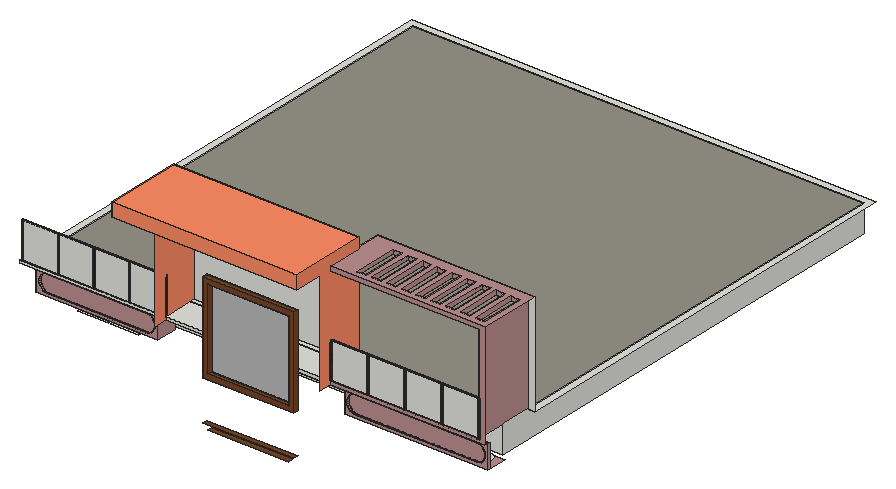
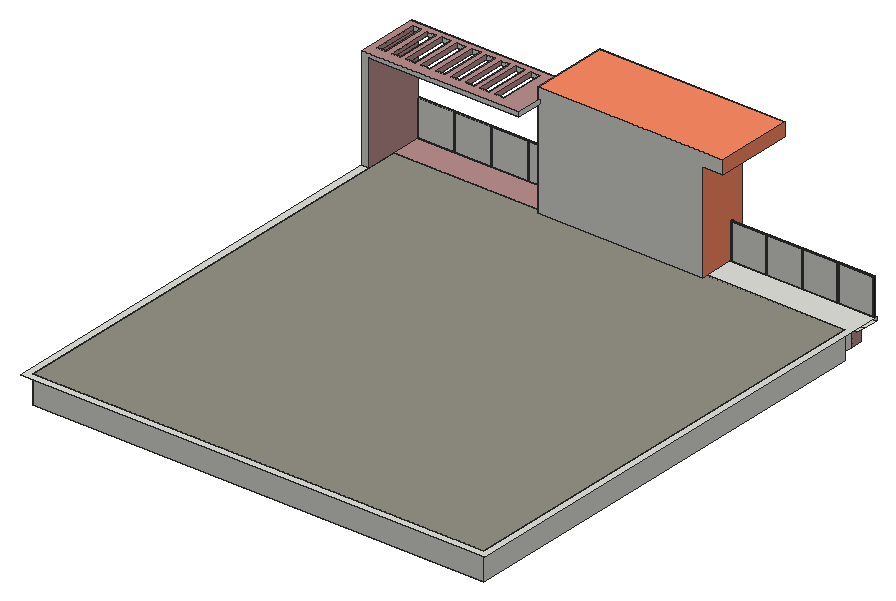
# SketchUp Ruby script. Lengths in inches.
U = 1.inch
M = Sketchup.active_model
def pt(a) = Geom::Point3d.new(a.map { |v| v * U })
def face(e, loops, mat)
  f = e.add_face(loops[0].map { |a| pt(a) })
  loops[1..].each { |l| e.add_face(l.map { |a| pt(a) }).erase! }
  f.material = f.back_material = mat if mat
  f
end
# faces: each face lists its corners as indices into pts; further lists are holes
def faces(e, pts, list, mat = nil) = list.each { |f| face(e, (f[0].is_a?(Array) ? f : [f]).map { |l| l.map { |i| pts[i] } }, mat) }
# xy, xz, yz: faces in a plane at the given z, y or x. An outline is a flat list of corners, or four numbers for a rectangle; further outlines are holes
def ring(l) = l.size == 4 ? [[l[0], l[1]], [l[2], l[1]], [l[2], l[3]], [l[0], l[3]]] : l.each_slice(2).to_a
def flat(e, list, mat, &to3) = list.each { |f| face(e, (f[0].is_a?(Array) ? f : [f]).map { |l| ring(l).map { |u, v| to3.(u, v) } }, mat) }
def xy(e, z, list, mat = nil) = flat(e, list, mat) { |x, y| [x, y, z] }
def xz(e, y, list, mat = nil) = flat(e, list, mat) { |x, z| [x, y, z] }
def yz(e, x, list, mat = nil) = flat(e, list, mat) { |y, z| [x, y, z] }
def lines(e, pts, list) = list.each { |a, b| e.add_line(pt(pts[a]), pt(pts[b])) }
# prism: a flat outline (further loops are holes) pulled along v
def prism(e, loops, v, mat = nil)
  f = face(e, loops, mat); d = Geom::Vector3d.new(v.map { |x| x * U })
  f.pushpull(f.normal.samedirection?(d) ? d.length : -d.length)
end
def box(e, o, s, mat = nil) = prism(e, [[o, [o[0] + s[0], o[1], o[2]], [o[0] + s[0], o[1] + s[1], o[2]], [o[0], o[1] + s[1], o[2]]]], [0, 0, s[2]], mat)
def at(x, y, z, deg = 0) = Geom::Transformation.translation(pt([x, y, z])) * Geom::Transformation.rotation(ORIGIN, Z_AXIS, deg.degrees)
def axes(o, x, y, z) = Geom::Transformation.new([*x, 0, *y, 0, *z, 0, *pt(o).to_a, 1])
def part(name) = M.definitions.add(name)
# library, detail: a bought-in or finely detailed component or shape, given as its bounding box
def library(name, o, s) = part(name).tap { |d| box(d.entities, o, s) }
def detail(e, o, s) = box(e.add_group.entities, o, s)
def put(e, d, t, mat = nil) = e.add_instance(d, t).tap { |i| i.material = mat if mat }
def group(e, t, mat = nil) = e.add_group.tap { |g| g.transformation = t; g.material = mat if mat }.entities
root = M.entities
M.materials.add("[0119_RosyBrown]").color = [188, 143, 143]
M.materials.add("[0136_Charcoal]").color = [35, 35, 35]
M.materials.add("[Color B03]").color = [255, 140, 101]
M.materials.add("[Formica Graystone]").color = [149, 146, 135]
M.materials.add("[Mirror 01]").color = [185, 185, 185]
M.materials.add("[Wood Veneer 01]").color = [120, 70, 37]
c1 = part("Group\#2")
box(c1.entities,[-152.36,0,0],[152.36,1.57,1.57])
c2 = part("Glass+Wall")
g1 = group(c2.entities,at(79.73,0,0))
g2 = group(g1,at(0,0,0))
g3 = group(g2,at(195.28,0,0),"[0136_Charcoal]")
box(g3,[-195.28,0,0],[195.28,1.57,1.57])
put(g2,c1,axes([1.57,0,116.54],[0,0,0.75452],[0,1,0],[-1,0,0]),"[0136_Charcoal]")
put(g2,c1,axes([50,0,116.54],[0,0,0.75452],[0,1,0],[-1,0,0]),"[0136_Charcoal]")
g4 = group(g2,at(195.28,0,115.75),"[0136_Charcoal]")
box(g4,[-195.28,0,0.79],[195.28,1.57,1.57])
put(g2,c1,axes([98.43,0,116.54],[0,0,0.75452],[0,1,0],[-1,0,0]),"[0136_Charcoal]")
put(g2,c1,axes([146.85,0,116.54],[0,0,0.75452],[0,1,0],[-1,0,0]),"[0136_Charcoal]")
put(g2,c1,axes([195.28,0,116.54],[0,0,0.75452],[0,1,0],[-1,0,0]),"[0136_Charcoal]")
g5 = group(g1,at(1.57,0.39,1.57))
box(g5,[0,0,0],[192.125,0.79,114.96])
xy(root,532.24,[[376.4,74.37,481.09,80.37]],"[Wood Veneer 01]")
xy(root,538.24,[[370.4,74.37,487.09,80.37]],"[Wood Veneer 01]")
xy(root,582.67,[[177.8,113.37,216.8,116.37],[219.92,113.37,255.8,116.37]])
xy(root,585.67,[[174.8,113.37,258.8,116.37]])
xy(root,590.49,[[370.4,74.37,487.09,80.37]],"[Wood Veneer 01]")
xy(root,595.17,[[593.68,113.37,630.53,116.37],[633.47,113.37,667.37,116.37]])
xy(root,596.49,[[376.4,74.37,481.09,80.37]],"[Wood Veneer 01]")
xy(root,598.17,[[590.68,113.37,670.37,116.37]])
xy(root,600,[[134.37,125.37,716.37,707.37]])
xy(root,602,[[540.59,89.37,725.37,92.37],[540.59,92.37,725.37,116.37]],"[0119_RosyBrown]")
xy(root,602.86,[[142.36,89.37,299.74,116.37]],"[0119_RosyBrown]")
xy(root,603.1875,[[291.4,94.48,293.11,94.75,294.69,95.46,296.04,96.55,297.05,97.95,297.67,99.56,297.85,101.28,297.58,102.99,296.88,104.57,295.79,105.91,294.39,106.93,292.78,107.55,291.06,107.73,289.35,107.46,287.77,106.76,286.42,105.67,285.41,104.27,284.79,102.65,284.61,100.93,284.88,99.23,285.58,97.65,286.67,96.3,288.07,95.28,289.68,94.66]])
xy(root,603.5,[[152.5,94.42,154.24,94.59,155.875,95.2,157.3,96.21,158.41,97.56,159.13,99.14,159.42,100.87,159.26,102.6,158.65,104.24,157.64,105.66,156.29,106.77,154.7,107.5,152.98,107.79,151.24,107.625,149.61,107.01,148.18,106,147.07,104.66,146.35,103.07,146.06,101.35,146.22,99.61,146.83,97.97,147.84,96.55,149.19,95.4375,150.78,94.71]])
xy(root,605,[[552.4375,89.37,712.19,92.37]],"[0119_RosyBrown]")
xy(root,605.86,[[153.74,89.37,288.27,92.37]])
xy(root,607.5,[[714.7,95.41,716.49,95.64,718.16,96.33,719.6,97.4375,720.7,98.875,721.4,100.55,721.63,102.34,721.4,104.14,720.7,105.8125,719.6,107.25,718.16,108.35,716.49,109.04,714.7,109.28,712.9,109.04,711.23,108.35,709.79,107.25,708.6875,105.8125,707.99,104.14,707.76,102.34,707.99,100.55,708.6875,98.875,709.79,97.4375,711.23,96.33,712.9,95.64]])
xy(root,621.125,[[548.88,95.41,550.68,95.64,552.35,96.33,553.79,97.4375,554.89,98.875,555.58,100.55,555.82,102.34,555.58,104.14,554.89,105.8125,553.79,107.25,552.35,108.35,550.68,109.04,548.88,109.28,547.09,109.04,545.41,108.35,543.98,107.25,542.875,105.8125,542.18,104.14,541.95,102.34,542.18,100.55,542.875,98.875,543.98,97.4375,545.41,96.33,547.09,95.64]])
xy(root,623,[[321.71,104.37,516.05,116.37]])
xy(root,629,[[153.74,89.37,288.27,92.37],[552.4375,89.37,712.19,92.37]],"[0119_RosyBrown]")
xy(root,632,[[125.37,85.68,142.36,104.37],[142.36,85.68,299.74,89.37],[299.74,85.68,312.71,89.37],[312.71,85.68,525.05,89.37],[525.05,85.68,725.37,89.37],
  [142.36,89.37,299.74,116.37],[299.74,89.37,312.71,116.37],[312.71,89.37,525.05,104.37],[525.05,89.37,540.59,116.37],[540.59,89.37,725.37,92.37],
  [125.37,104.37,142.36,116.37]])
xy(root,636,[[125.37,85.68,312.71,85.68,312.71,125.37,134.37,125.37,134.37,707.37,716.37,707.37,716.37,165.62,725.37,165.62,725.37,716.37,125.37,716.37],[312.71,85.68,525.05,125.37],[312.71,125.37,525.05,131.99]])
xy(root,636,[[525.05,85.68,716.37,125.37]],"[0119_RosyBrown]")
xy(root,636,[[134.37,125.37,312.71,125.37,312.71,131.99,525.05,131.99,525.05,125.37,716.37,125.37,716.37,707.37,134.37,707.37]],"[Formica Graystone]")
xy(root,701.18,[[376.4,74.37,481.09,80.37]])
xy(root,707.18,[[370.4,74.37,487.09,80.37]],"[Wood Veneer 01]")
xy(root,763.25,[[716.37,94.07,717.24,151.69]])
xy(root,763.25,[[[522.43,85.68,522.43,165.62,716.37,165.62,716.37,151.69,705.8,151.69,705.8,94.07,716.37,94.07,716.37,85.68],[553.3,94.07,564.74,151.69],[572.36,94.07,583.8,151.69],[591.43,94.07,602.86,151.69],[610.49,94.07,621.93,151.69],[629.55,94.07,640.99,151.69],[648.61,94.07,660.05,151.69],[667.68,94.07,679.11,151.69],[686.74,94.07,698.18,151.69]]],"[0119_RosyBrown]")
xy(root,764.5625,[[286.02,32.37,286.02,131.99,312.71,131.99,312.71,68.37,321.71,68.37,321.71,80.37,516.05,80.37,516.05,68.37,525.05,68.37,525.05,32.37]],"[Color B03]")
xy(root,768.6875,[[[522.43,85.68,725.37,165.62],[553.3,94.07,564.74,151.69],[572.36,94.07,583.8,151.69],[591.43,94.07,602.86,151.69],[610.49,94.07,621.93,151.69],[629.55,94.07,640.99,151.69],[648.61,94.07,660.05,151.69],[667.68,94.07,679.11,151.69],[686.74,94.07,698.18,151.69],[705.8,94.07,717.24,151.69]]],"[0119_RosyBrown]")
xy(root,782.0625,[[286.02,32.37,525.05,131.99]],"[Color B03]")
xz(root,32.37,[[286.02,764.5625,525.05,782.0625]],"[Color B03]")
xz(root,74.37,[[[370.4,590.49,487.09,707.18],[376.4,596.49,481.09,701.18]]],"[Wood Veneer 01]")
xz(root,80.37,[[[370.4,590.49,487.09,707.18],[376.4,596.49,481.09,701.18]]])
xz(root,80.37,[[376.4,596.49,481.09,701.18]],"[Mirror 01]")
xz(root,85.68,[[125.37,632,312.71,636],[312.71,632,525.05,636]])
xz(root,85.68,[[525.05,632,725.37,632,725.37,768.6875,522.43,768.6875,522.43,763.25,716.37,763.25,716.37,636,525.05,636]],"[0119_RosyBrown]")
xz(root,89.37,[[[540.59,602,725.37,632],[552.4375,605,550,606.05,547.84,607.59,546.04,609.55,544.7,611.84,543.875,614.36,543.59,617,543.875,619.64,544.7,622.16,546.04,624.45,547.84,626.41,550,627.95,552.4375,629,712.19,629,714.93,628.21,717.4,626.81,719.48,624.87,721.06,622.5,722.03,619.83,722.37,617,722.03,614.18,721.06,611.5,719.48,609.13,717.4,607.19,714.93,605.79,712.19,605]],[[142.36,602.86,299.74,632],[153.74,605.86,151.66,607.08,149.85,608.67,148.36,610.57,147.27,612.72,146.59,615.03,146.36,617.43,146.59,619.83,147.27,622.14,148.36,624.29,149.85,626.19,151.66,627.78,153.74,629,288.27,629,290.4,627.8125,292.25,626.24,293.77,624.34,294.9,622.18,295.6,619.85,295.83,617.43,295.6,615.01,294.9,612.68,293.77,610.52,292.25,608.62,290.4,607.05,288.27,605.86]]],"[0119_RosyBrown]")
xz(root,92.37,[[[540.59,602,725.37,632],[552.4375,605,712.19,605,714.93,605.79,717.4,607.19,719.48,609.13,721.06,611.5,722.03,614.18,722.37,617,722.03,619.83,721.06,622.5,719.48,624.87,717.4,626.81,714.93,628.21,712.19,629,552.4375,629,550,627.95,547.84,626.41,546.04,624.45,544.7,622.16,543.875,619.64,543.59,617,543.875,614.36,544.7,611.84,546.04,609.55,547.84,607.59,550,606.05]]])
xz(root,92.37,[[552.4375,605,712.19,605,714.93,605.79,717.4,607.19,719.48,609.13,721.06,611.5,722.03,614.18,722.37,617,722.03,619.83,721.06,622.5,719.48,624.87,717.4,626.81,714.93,628.21,712.19,629,552.4375,629,550,627.95,547.84,626.41,546.04,624.45,544.7,622.16,543.875,619.64,543.59,617,543.875,614.36,544.7,611.84,546.04,609.55,547.84,607.59,550,606.05],[153.74,605.86,288.27,605.86,290.4,607.05,292.25,608.62,293.77,610.52,294.9,612.68,295.6,615.01,295.83,617.43,295.6,619.85,294.9,622.18,293.77,624.34,292.25,626.24,290.4,627.8125,288.27,629,153.74,629,151.66,627.78,149.85,626.19,148.36,624.29,147.27,622.14,146.59,619.83,146.36,617.43,146.59,615.03,147.27,612.72,148.36,610.57,149.85,608.67,151.66,607.08]],"[0119_RosyBrown]")
xz(root,94.07,[[553.3,763.25,564.74,768.6875],[572.36,763.25,583.8,768.6875],[591.43,763.25,602.86,768.6875],[610.49,763.25,621.93,768.6875],[629.55,763.25,640.99,768.6875],
  [648.61,763.25,660.05,768.6875],[667.68,763.25,679.11,768.6875],[686.74,763.25,698.18,768.6875],[705.8,763.25,717.24,768.6875]])
xz(root,125.37,[[134.37,600,716.37,636]])
xz(root,131.99,[[312.71,636,312.71,764.5625,286.02,764.5625,286.02,782.0625,525.05,782.0625,525.05,636]])
xz(root,151.69,[[553.3,763.25,564.74,768.6875],[572.36,763.25,583.8,768.6875],[591.43,763.25,602.86,768.6875],[610.49,763.25,621.93,768.6875],[629.55,763.25,640.99,768.6875],
  [648.61,763.25,660.05,768.6875],[667.68,763.25,679.11,768.6875],[686.74,763.25,698.18,768.6875],[705.8,763.25,717.24,768.6875]],"[0119_RosyBrown]")
xz(root,165.62,[[716.37,636,716.37,763.25,522.43,763.25,522.43,768.6875,725.37,768.6875,725.37,636]])
xz(root,707.37,[[134.37,600,716.37,636]])
yz(root,134.37,[[125.37,600,707.37,636]])
yz(root,142.36,[[104.37,602.86,113.37,632],[113.37,602.86,116.37,632]])
yz(root,142.36,[[89.37,602.86,104.37,632]],"[0119_RosyBrown]")
yz(root,286.02,[[32.37,764.5625,131.99,782.0625]],"[Color B03]")
yz(root,299.74,[[89.37,602.86,116.37,632]],"[0119_RosyBrown]")
yz(root,312.71,[[68.37,632,68.37,764.5625,131.99,764.5625,131.99,636,85.68,636,85.68,632]],"[Color B03]")
yz(root,370.4,[[74.37,590.49,80.37,707.18]],"[Wood Veneer 01]")
yz(root,376.4,[[74.37,596.49,80.37,701.18]],"[Wood Veneer 01]")
yz(root,481.09,[[74.37,596.49,80.37,701.18]],"[Wood Veneer 01]")
yz(root,487.09,[[74.37,590.49,80.37,707.18]],"[Wood Veneer 01]")
yz(root,522.43,[[85.68,763.25,165.62,768.6875]])
yz(root,525.05,[[68.37,632,85.68,632,85.68,636,131.99,636,131.99,782.0625,32.37,782.0625,32.37,764.5625,68.37,764.5625]],"[Color B03]")
yz(root,540.59,[[89.37,602,92.37,632],[92.37,602,116.37,632]],"[0119_RosyBrown]")
yz(root,553.3,[[94.07,763.25,151.69,768.6875]],"[0119_RosyBrown]")
yz(root,564.74,[[94.07,763.25,151.69,768.6875]],"[0119_RosyBrown]")
yz(root,572.36,[[94.07,763.25,151.69,768.6875]],"[0119_RosyBrown]")
yz(root,583.8,[[94.07,763.25,151.69,768.6875]],"[0119_RosyBrown]")
yz(root,591.43,[[94.07,763.25,151.69,768.6875]],"[0119_RosyBrown]")
yz(root,602.86,[[94.07,763.25,151.69,768.6875]],"[0119_RosyBrown]")
yz(root,610.49,[[94.07,763.25,151.69,768.6875]],"[0119_RosyBrown]")
yz(root,621.93,[[94.07,763.25,151.69,768.6875]],"[0119_RosyBrown]")
yz(root,629.55,[[94.07,763.25,151.69,768.6875]],"[0119_RosyBrown]")
yz(root,640.99,[[94.07,763.25,151.69,768.6875]],"[0119_RosyBrown]")
yz(root,648.61,[[94.07,763.25,151.69,768.6875]],"[0119_RosyBrown]")
yz(root,660.05,[[94.07,763.25,151.69,768.6875]],"[0119_RosyBrown]")
yz(root,667.68,[[94.07,763.25,151.69,768.6875]],"[0119_RosyBrown]")
yz(root,679.11,[[94.07,763.25,151.69,768.6875]],"[0119_RosyBrown]")
yz(root,686.74,[[94.07,763.25,151.69,768.6875]],"[0119_RosyBrown]")
yz(root,698.18,[[94.07,763.25,151.69,768.6875]],"[0119_RosyBrown]")
yz(root,705.8,[[94.07,763.25,151.69,768.6875]],"[0119_RosyBrown]")
yz(root,716.37,[[125.37,600,707.37,636]])
yz(root,716.37,[[85.68,636,165.62,763.25]],"[0119_RosyBrown]")
yz(root,717.24,[[94.07,763.25,151.69,768.6875]],"[0119_RosyBrown]")
yz(root,725.37,[[89.37,602,92.37,632]],"[0119_RosyBrown]")
p = [[552.4375,92.37,605],[550,92.37,606.05],[550,89.37,606.05],[552.4375,89.37,605],[714.93,92.37,605.79],[712.19,92.37,605],
  [712.19,89.37,605],[714.93,89.37,605.79],[717.4,92.37,607.19],[717.4,89.37,607.19],[153.74,92.37,605.86],[151.66,92.37,607.08],
  [151.66,89.37,607.08],[153.74,89.37,605.86],[290.4,92.37,607.05],[288.27,92.37,605.86],[288.27,89.37,605.86],[290.4,89.37,607.05],
  [547.84,92.37,607.59],[547.84,89.37,607.59],[292.25,92.37,608.62],[292.25,89.37,608.62],[149.85,92.37,608.67],[149.85,89.37,608.67],
  [719.48,92.37,609.13],[719.48,89.37,609.13],[546.04,92.37,609.55],[546.04,89.37,609.55],[293.77,92.37,610.52],[293.77,89.37,610.52],
  [148.36,92.37,610.57],[148.36,89.37,610.57],[721.06,92.37,611.5],[721.06,89.37,611.5],[544.7,92.37,611.84],[544.7,89.37,611.84],
  [294.9,92.37,612.68],[294.9,89.37,612.68],[147.27,92.37,612.72],[147.27,89.37,612.72],[722.03,92.37,614.18],[722.03,89.37,614.18],
  [543.875,92.37,614.36],[543.875,89.37,614.36],[146.59,92.37,615.03],[146.59,89.37,615.03],[295.6,92.37,615.01],[295.6,89.37,615.01],
  [722.37,92.37,617],[722.37,89.37,617],[543.59,92.37,617],[543.59,89.37,617],[146.36,92.37,617.43],[146.36,89.37,617.43],
  [295.83,92.37,617.43],[295.83,89.37,617.43],[543.875,92.37,619.64],[543.875,89.37,619.64],[722.03,92.37,619.83],[722.03,89.37,619.83],
  [146.59,92.37,619.83],[146.59,89.37,619.83],[295.6,92.37,619.85],[295.6,89.37,619.85],[544.7,92.37,622.16],[544.7,89.37,622.16],
  [147.27,92.37,622.14],[147.27,89.37,622.14],[721.06,92.37,622.5],[721.06,89.37,622.5],[294.9,92.37,622.18],[294.9,89.37,622.18],
  [148.36,92.37,624.29],[148.36,89.37,624.29],[293.77,92.37,624.34],[293.77,89.37,624.34],[546.04,92.37,624.45],[546.04,89.37,624.45],
  [719.48,92.37,624.87],[719.48,89.37,624.87],[149.85,92.37,626.19],[149.85,89.37,626.19],[292.25,92.37,626.24],[292.25,89.37,626.24],
  [547.84,92.37,626.41],[547.84,89.37,626.41],[717.4,92.37,626.81],[717.4,89.37,626.81],[151.66,92.37,627.78],[151.66,89.37,627.78],
  [290.4,92.37,627.8125],[290.4,89.37,627.8125],[550,92.37,627.95],[550,89.37,627.95],[714.93,92.37,628.21],[714.93,89.37,628.21],
  [153.74,92.37,629],[153.74,89.37,629],[288.27,92.37,629],[288.27,89.37,629],[552.4375,92.37,629],[552.4375,89.37,629],
  [712.19,92.37,629],[712.19,89.37,629],[142.36,116.37,632],[142.36,116.37,636],[299.74,116.37,632],[299.74,116.37,636],
  [540.59,116.37,632],[540.59,116.37,632.75]]
faces(root,p,[[0,1,2,3],[4,5,6,7],[8,4,7,9],[10,11,12,13],[14,15,16,17],[1,18,19,2],[20,14,17,21],[11,22,23,12],
  [24,8,9,25],[18,26,27,19],[28,20,21,29],[22,30,31,23],[32,24,25,33],[26,34,35,27],[36,28,29,37],[30,38,39,31],
  [40,32,33,41],[34,42,43,35],[38,44,45,39],[46,36,37,47],[48,40,41,49],[42,50,51,43],[44,52,53,45],[54,46,47,55],
  [50,56,57,51],[58,48,49,59],[52,60,61,53],[62,54,55,63],[56,64,65,57],[60,66,67,61],[68,58,59,69],[70,62,63,71],
  [66,72,73,67],[74,70,71,75],[64,76,77,65],[78,68,69,79],[72,80,81,73],[82,74,75,83],[76,84,85,77],[86,78,79,87],
  [80,88,89,81],[90,82,83,91],[84,92,93,85],[94,86,87,95],[88,96,97,89],[98,90,91,99],[92,100,101,93],[102,94,95,103]],"[0119_RosyBrown]")
lines(root,p,[[104,105],[106,107],[108,109]])
put(root,c2,axes([51.44,87.07,635.37],[0.95007,0,0],[0,-0.882,0],[0,0,0.4032]))
put(root,c2,axes([446.34,87.07,636],[0.98725,0,0],[0,-0.882,0],[0,0,0.4032]))
